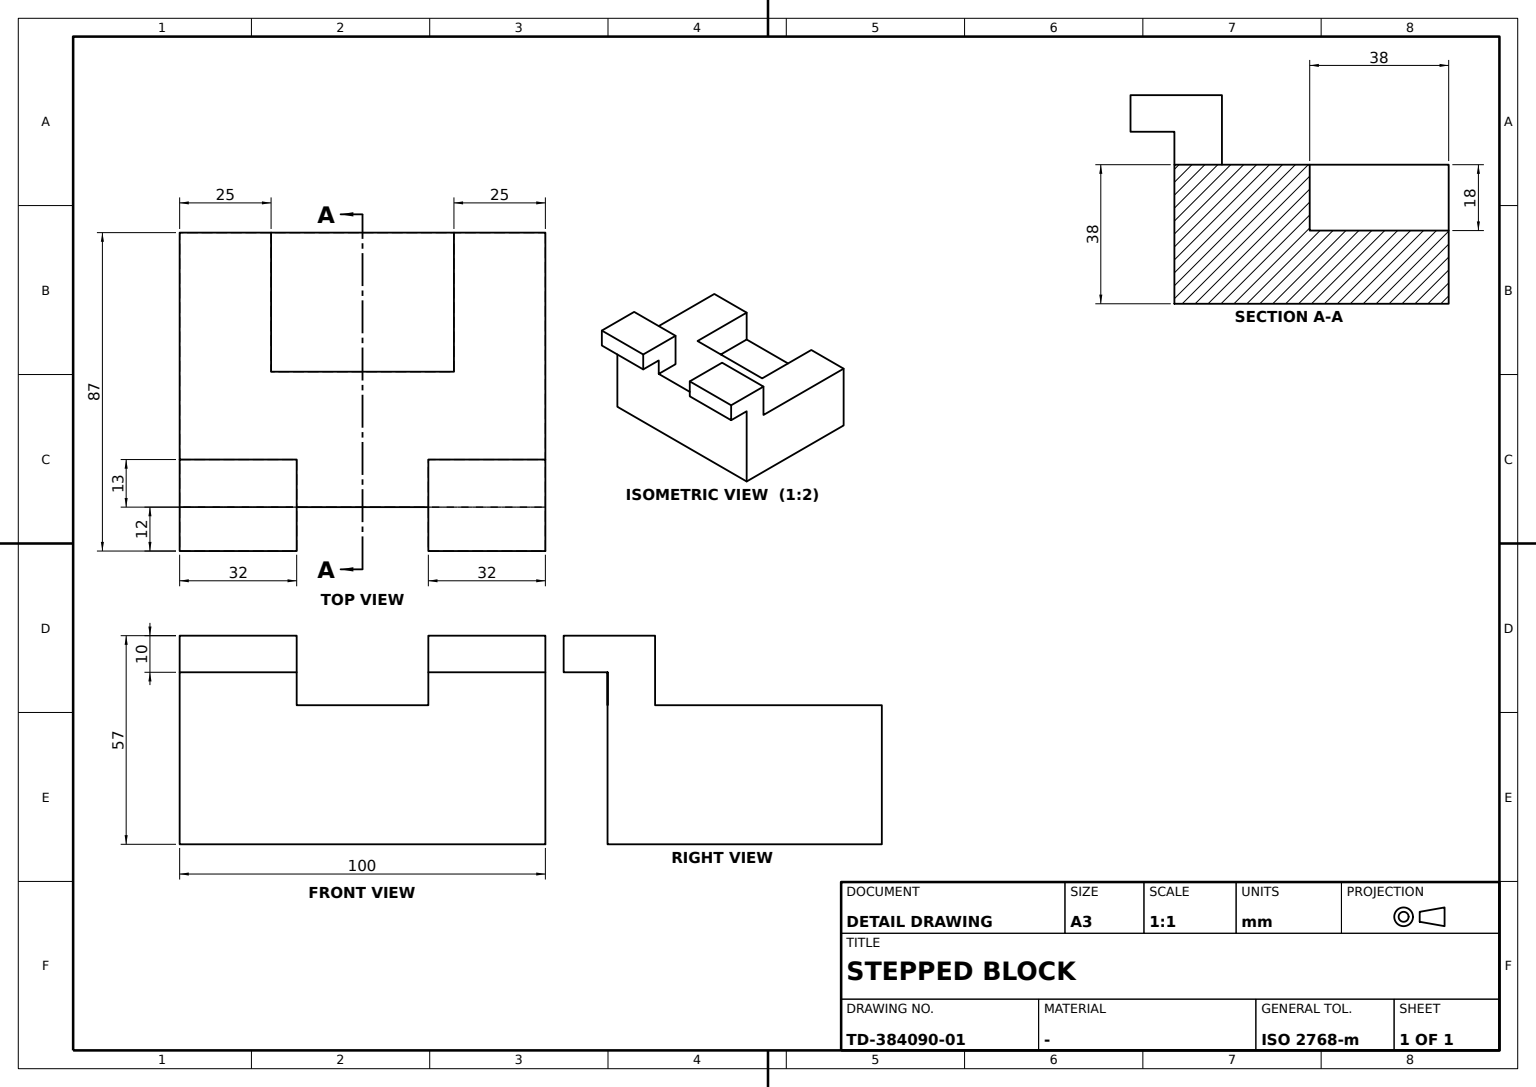
ISO-10303-21;
HEADER;
FILE_DESCRIPTION((''),'2;1');
FILE_NAME('','',(''),(''),'','','');
FILE_SCHEMA(('AUTOMOTIVE_DESIGN'));
ENDSEC;
DATA;
#1=APPLICATION_CONTEXT('');
#2=PRODUCT_CONTEXT('',#1,'mechanical');
#3=PRODUCT('','','',(#2));
#4=PRODUCT_DEFINITION_FORMATION('','',#3);
#5=PRODUCT_DEFINITION_CONTEXT('',#1,'design');
#6=PRODUCT_DEFINITION('','',#4,#5);
#7=PRODUCT_DEFINITION_SHAPE('','',#6);
#8=(LENGTH_UNIT()NAMED_UNIT(*)SI_UNIT(.MILLI.,.METRE.));
#9=(NAMED_UNIT(*)PLANE_ANGLE_UNIT()SI_UNIT($,.RADIAN.));
#10=(NAMED_UNIT(*)SI_UNIT($,.STERADIAN.)SOLID_ANGLE_UNIT());
#11=UNCERTAINTY_MEASURE_WITH_UNIT(LENGTH_MEASURE(0.005),#8,'distance_accuracy_value','');
#12=(GEOMETRIC_REPRESENTATION_CONTEXT(3)GLOBAL_UNCERTAINTY_ASSIGNED_CONTEXT((#11))GLOBAL_UNIT_ASSIGNED_CONTEXT((#8,#9,#10))REPRESENTATION_CONTEXT('',''));
#13=CARTESIAN_POINT('',(-50.,-49.5,57.));
#14=VERTEX_POINT('',#13);
#15=CARTESIAN_POINT('',(-50.,-49.5,47.));
#16=VERTEX_POINT('',#15);
#17=DIRECTION('',(0.,0.,-1.));
#18=VECTOR('',#17,1000.);
#19=LINE('',#13,#18);
#20=EDGE_CURVE('',#14,#16,#19,.T.);
#21=ORIENTED_EDGE('',*,*,#20,.T.);
#22=CARTESIAN_POINT('',(-18.,-49.5,47.));
#23=VERTEX_POINT('',#22);
#24=CARTESIAN_POINT('',(50.,-49.5,47.));
#25=DIRECTION('',(1.,0.,0.));
#26=VECTOR('',#25,1000.);
#27=LINE('',#24,#26);
#28=EDGE_CURVE('',#16,#23,#27,.T.);
#29=ORIENTED_EDGE('',*,*,#28,.T.);
#30=CARTESIAN_POINT('',(-18.,-49.5,57.));
#31=VERTEX_POINT('',#30);
#32=LINE('',#30,#18);
#33=EDGE_CURVE('',#31,#23,#32,.T.);
#34=ORIENTED_EDGE('',*,*,#33,.F.);
#35=CARTESIAN_POINT('',(50.,-49.5,57.));
#36=LINE('',#35,#26);
#37=EDGE_CURVE('',#14,#31,#36,.T.);
#38=ORIENTED_EDGE('',*,*,#37,.F.);
#39=EDGE_LOOP('',(#21,#29,#34,#38));
#40=FACE_BOUND('',#39,.T.);
#41=DIRECTION('',(0.,1.,0.));
#42=AXIS2_PLACEMENT_3D('',#35,#41,#17);
#43=PLANE('',#42);
#44=ADVANCED_FACE('',(#40),#43,.F.);
#45=CARTESIAN_POINT('',(-50.,-37.5,47.));
#46=VERTEX_POINT('',#45);
#47=CARTESIAN_POINT('',(-18.,-37.5,47.));
#48=VERTEX_POINT('',#47);
#49=CARTESIAN_POINT('',(50.,-37.5,47.));
#50=LINE('',#49,#26);
#51=EDGE_CURVE('',#46,#48,#50,.T.);
#52=ORIENTED_EDGE('',*,*,#51,.T.);
#53=VECTOR('',#41,1000.);
#54=LINE('',#22,#53);
#55=EDGE_CURVE('',#23,#48,#54,.T.);
#56=ORIENTED_EDGE('',*,*,#55,.F.);
#57=ORIENTED_EDGE('',*,*,#28,.F.);
#58=LINE('',#15,#53);
#59=EDGE_CURVE('',#16,#46,#58,.T.);
#60=ORIENTED_EDGE('',*,*,#59,.T.);
#61=EDGE_LOOP('',(#52,#56,#57,#60));
#62=FACE_BOUND('',#61,.T.);
#63=DIRECTION('',(0.,0.,1.));
#64=AXIS2_PLACEMENT_3D('',#24,#63,#41);
#65=PLANE('',#64);
#66=ADVANCED_FACE('',(#62),#65,.F.);
#67=CARTESIAN_POINT('',(-50.,-37.5,0.));
#68=VERTEX_POINT('',#67);
#69=VECTOR('',#63,1000.);
#70=LINE('',#67,#69);
#71=EDGE_CURVE('',#68,#46,#70,.T.);
#72=ORIENTED_EDGE('',*,*,#71,.F.);
#73=CARTESIAN_POINT('',(50.,-37.5,0.));
#74=VERTEX_POINT('',#73);
#75=CARTESIAN_POINT('',(0.,-37.5,0.));
#76=DIRECTION('',(-1.,0.,0.));
#77=VECTOR('',#76,1000.);
#78=LINE('',#75,#77);
#79=EDGE_CURVE('',#74,#68,#78,.T.);
#80=ORIENTED_EDGE('',*,*,#79,.F.);
#81=VERTEX_POINT('',#49);
#82=LINE('',#73,#69);
#83=EDGE_CURVE('',#74,#81,#82,.T.);
#84=ORIENTED_EDGE('',*,*,#83,.T.);
#85=CARTESIAN_POINT('',(18.,-37.5,47.));
#86=VERTEX_POINT('',#85);
#87=LINE('',#49,#77);
#88=EDGE_CURVE('',#81,#86,#87,.T.);
#89=ORIENTED_EDGE('',*,*,#88,.T.);
#90=CARTESIAN_POINT('',(18.,-37.5,38.));
#91=VERTEX_POINT('',#90);
#92=CARTESIAN_POINT('',(18.,-37.5,0.));
#93=LINE('',#92,#18);
#94=EDGE_CURVE('',#86,#91,#93,.T.);
#95=ORIENTED_EDGE('',*,*,#94,.T.);
#96=CARTESIAN_POINT('',(-18.,-37.5,38.));
#97=VERTEX_POINT('',#96);
#98=CARTESIAN_POINT('',(0.,-37.5,38.));
#99=LINE('',#98,#77);
#100=EDGE_CURVE('',#91,#97,#99,.T.);
#101=ORIENTED_EDGE('',*,*,#100,.T.);
#102=CARTESIAN_POINT('',(-18.,-37.5,0.));
#103=LINE('',#102,#18);
#104=EDGE_CURVE('',#48,#97,#103,.T.);
#105=ORIENTED_EDGE('',*,*,#104,.F.);
#106=ORIENTED_EDGE('',*,*,#51,.F.);
#107=EDGE_LOOP('',(#72,#80,#84,#89,#95,#101,#105,#106));
#108=FACE_BOUND('',#107,.T.);
#109=AXIS2_PLACEMENT_3D('',#73,#41,#76);
#110=PLANE('',#109);
#111=ADVANCED_FACE('',(#108),#110,.F.);
#112=CARTESIAN_POINT('',(18.,-24.5,57.));
#113=VERTEX_POINT('',#112);
#114=CARTESIAN_POINT('',(18.,-49.5,57.));
#115=VERTEX_POINT('',#114);
#116=DIRECTION('',(0.,-1.,0.));
#117=VECTOR('',#116,1000.);
#118=LINE('',#112,#117);
#119=EDGE_CURVE('',#113,#115,#118,.T.);
#120=ORIENTED_EDGE('',*,*,#119,.T.);
#121=VERTEX_POINT('',#35);
#122=LINE('',#35,#77);
#123=EDGE_CURVE('',#121,#115,#122,.T.);
#124=ORIENTED_EDGE('',*,*,#123,.F.);
#125=CARTESIAN_POINT('',(50.,-24.5,57.));
#126=VERTEX_POINT('',#125);
#127=CARTESIAN_POINT('',(50.,37.5,57.));
#128=LINE('',#127,#117);
#129=EDGE_CURVE('',#126,#121,#128,.T.);
#130=ORIENTED_EDGE('',*,*,#129,.F.);
#131=LINE('',#125,#77);
#132=EDGE_CURVE('',#126,#113,#131,.T.);
#133=ORIENTED_EDGE('',*,*,#132,.T.);
#134=EDGE_LOOP('',(#120,#124,#130,#133));
#135=FACE_BOUND('',#134,.T.);
#136=AXIS2_PLACEMENT_3D('',#125,#17,#116);
#137=PLANE('',#136);
#138=ADVANCED_FACE('',(#135),#137,.F.);
#139=CARTESIAN_POINT('',(25.,-0.5,38.));
#140=VERTEX_POINT('',#139);
#141=CARTESIAN_POINT('',(25.,-0.5,20.));
#142=VERTEX_POINT('',#141);
#143=LINE('',#139,#18);
#144=EDGE_CURVE('',#140,#142,#143,.T.);
#145=ORIENTED_EDGE('',*,*,#144,.T.);
#146=CARTESIAN_POINT('',(-25.,-0.5,20.));
#147=VERTEX_POINT('',#146);
#148=LINE('',#146,#26);
#149=EDGE_CURVE('',#147,#142,#148,.T.);
#150=ORIENTED_EDGE('',*,*,#149,.F.);
#151=CARTESIAN_POINT('',(-25.,-0.5,38.));
#152=VERTEX_POINT('',#151);
#153=LINE('',#151,#18);
#154=EDGE_CURVE('',#152,#147,#153,.T.);
#155=ORIENTED_EDGE('',*,*,#154,.F.);
#156=LINE('',#151,#26);
#157=EDGE_CURVE('',#152,#140,#156,.T.);
#158=ORIENTED_EDGE('',*,*,#157,.T.);
#159=EDGE_LOOP('',(#145,#150,#155,#158));
#160=FACE_BOUND('',#159,.T.);
#161=AXIS2_PLACEMENT_3D('',#151,#41,#25);
#162=PLANE('',#161);
#163=ADVANCED_FACE('',(#160),#162,.T.);
#164=CARTESIAN_POINT('',(25.,37.5,38.));
#165=VERTEX_POINT('',#164);
#166=LINE('',#139,#53);
#167=EDGE_CURVE('',#140,#165,#166,.T.);
#168=ORIENTED_EDGE('',*,*,#167,.F.);
#169=ORIENTED_EDGE('',*,*,#157,.F.);
#170=CARTESIAN_POINT('',(-25.,37.5,38.));
#171=VERTEX_POINT('',#170);
#172=LINE('',#170,#117);
#173=EDGE_CURVE('',#171,#152,#172,.T.);
#174=ORIENTED_EDGE('',*,*,#173,.F.);
#175=CARTESIAN_POINT('',(-50.,37.5,38.));
#176=VERTEX_POINT('',#175);
#177=CARTESIAN_POINT('',(0.,37.5,38.));
#178=LINE('',#177,#26);
#179=EDGE_CURVE('',#176,#171,#178,.T.);
#180=ORIENTED_EDGE('',*,*,#179,.F.);
#181=CARTESIAN_POINT('',(-50.,-24.5,38.));
#182=VERTEX_POINT('',#181);
#183=CARTESIAN_POINT('',(-50.,0.,38.));
#184=LINE('',#183,#53);
#185=EDGE_CURVE('',#182,#176,#184,.T.);
#186=ORIENTED_EDGE('',*,*,#185,.F.);
#187=CARTESIAN_POINT('',(-18.,-24.5,38.));
#188=VERTEX_POINT('',#187);
#189=CARTESIAN_POINT('',(0.,-24.5,38.));
#190=LINE('',#189,#26);
#191=EDGE_CURVE('',#182,#188,#190,.T.);
#192=ORIENTED_EDGE('',*,*,#191,.T.);
#193=CARTESIAN_POINT('',(-18.,0.,38.));
#194=LINE('',#193,#53);
#195=EDGE_CURVE('',#97,#188,#194,.T.);
#196=ORIENTED_EDGE('',*,*,#195,.F.);
#197=ORIENTED_EDGE('',*,*,#100,.F.);
#198=CARTESIAN_POINT('',(18.,-24.5,38.));
#199=VERTEX_POINT('',#198);
#200=CARTESIAN_POINT('',(18.,0.,38.));
#201=LINE('',#200,#53);
#202=EDGE_CURVE('',#91,#199,#201,.T.);
#203=ORIENTED_EDGE('',*,*,#202,.T.);
#204=CARTESIAN_POINT('',(50.,-24.5,38.));
#205=VERTEX_POINT('',#204);
#206=LINE('',#204,#77);
#207=EDGE_CURVE('',#205,#199,#206,.T.);
#208=ORIENTED_EDGE('',*,*,#207,.F.);
#209=CARTESIAN_POINT('',(50.,37.5,38.));
#210=VERTEX_POINT('',#209);
#211=CARTESIAN_POINT('',(50.,0.,38.));
#212=LINE('',#211,#117);
#213=EDGE_CURVE('',#210,#205,#212,.T.);
#214=ORIENTED_EDGE('',*,*,#213,.F.);
#215=EDGE_CURVE('',#165,#210,#178,.T.);
#216=ORIENTED_EDGE('',*,*,#215,.F.);
#217=EDGE_LOOP('',(#168,#169,#174,#180,#186,#192,#196,#197,#203,#208,#214,#216));
#218=FACE_BOUND('',#217,.T.);
#219=CARTESIAN_POINT('',(0.,0.,38.));
#220=AXIS2_PLACEMENT_3D('',#219,#63,#25);
#221=PLANE('',#220);
#222=ADVANCED_FACE('',(#218),#221,.T.);
#223=ORIENTED_EDGE('',*,*,#173,.T.);
#224=ORIENTED_EDGE('',*,*,#154,.T.);
#225=CARTESIAN_POINT('',(-25.,37.5,20.));
#226=VERTEX_POINT('',#225);
#227=LINE('',#225,#117);
#228=EDGE_CURVE('',#226,#147,#227,.T.);
#229=ORIENTED_EDGE('',*,*,#228,.F.);
#230=LINE('',#170,#18);
#231=EDGE_CURVE('',#171,#226,#230,.T.);
#232=ORIENTED_EDGE('',*,*,#231,.F.);
#233=EDGE_LOOP('',(#223,#224,#229,#232));
#234=FACE_BOUND('',#233,.T.);
#235=AXIS2_PLACEMENT_3D('',#170,#25,#116);
#236=PLANE('',#235);
#237=ADVANCED_FACE('',(#234),#236,.T.);
#238=CARTESIAN_POINT('',(25.,37.5,20.));
#239=VERTEX_POINT('',#238);
#240=LINE('',#141,#53);
#241=EDGE_CURVE('',#142,#239,#240,.T.);
#242=ORIENTED_EDGE('',*,*,#241,.F.);
#243=ORIENTED_EDGE('',*,*,#144,.F.);
#244=ORIENTED_EDGE('',*,*,#167,.T.);
#245=CARTESIAN_POINT('',(25.,37.5,0.));
#246=LINE('',#245,#18);
#247=EDGE_CURVE('',#165,#239,#246,.T.);
#248=ORIENTED_EDGE('',*,*,#247,.T.);
#249=EDGE_LOOP('',(#242,#243,#244,#248));
#250=FACE_BOUND('',#249,.T.);
#251=AXIS2_PLACEMENT_3D('',#139,#76,#41);
#252=PLANE('',#251);
#253=ADVANCED_FACE('',(#250),#252,.T.);
#254=ORIENTED_EDGE('',*,*,#129,.T.);
#255=VERTEX_POINT('',#24);
#256=CARTESIAN_POINT('',(50.,-49.5,0.));
#257=LINE('',#256,#18);
#258=EDGE_CURVE('',#121,#255,#257,.T.);
#259=ORIENTED_EDGE('',*,*,#258,.T.);
#260=CARTESIAN_POINT('',(50.,37.5,47.));
#261=LINE('',#260,#53);
#262=EDGE_CURVE('',#255,#81,#261,.T.);
#263=ORIENTED_EDGE('',*,*,#262,.T.);
#264=ORIENTED_EDGE('',*,*,#83,.F.);
#265=CARTESIAN_POINT('',(50.,37.5,0.));
#266=VERTEX_POINT('',#265);
#267=CARTESIAN_POINT('',(50.,0.,0.));
#268=LINE('',#267,#117);
#269=EDGE_CURVE('',#266,#74,#268,.T.);
#270=ORIENTED_EDGE('',*,*,#269,.F.);
#271=LINE('',#265,#69);
#272=EDGE_CURVE('',#266,#210,#271,.T.);
#273=ORIENTED_EDGE('',*,*,#272,.T.);
#274=ORIENTED_EDGE('',*,*,#213,.T.);
#275=CARTESIAN_POINT('',(50.,-24.5,0.));
#276=LINE('',#275,#69);
#277=EDGE_CURVE('',#205,#126,#276,.T.);
#278=ORIENTED_EDGE('',*,*,#277,.T.);
#279=EDGE_LOOP('',(#254,#259,#263,#264,#270,#273,#274,#278));
#280=FACE_BOUND('',#279,.T.);
#281=AXIS2_PLACEMENT_3D('',#265,#76,#116);
#282=PLANE('',#281);
#283=ADVANCED_FACE('',(#280),#282,.F.);
#284=CARTESIAN_POINT('',(-50.,-24.5,57.));
#285=VERTEX_POINT('',#284);
#286=LINE('',#284,#117);
#287=EDGE_CURVE('',#285,#14,#286,.T.);
#288=ORIENTED_EDGE('',*,*,#287,.T.);
#289=ORIENTED_EDGE('',*,*,#37,.T.);
#290=CARTESIAN_POINT('',(-18.,-24.5,57.));
#291=VERTEX_POINT('',#290);
#292=LINE('',#290,#117);
#293=EDGE_CURVE('',#291,#31,#292,.T.);
#294=ORIENTED_EDGE('',*,*,#293,.F.);
#295=LINE('',#125,#26);
#296=EDGE_CURVE('',#285,#291,#295,.T.);
#297=ORIENTED_EDGE('',*,*,#296,.F.);
#298=EDGE_LOOP('',(#288,#289,#294,#297));
#299=FACE_BOUND('',#298,.T.);
#300=ADVANCED_FACE('',(#299),#137,.F.);
#301=LINE('',#181,#69);
#302=EDGE_CURVE('',#182,#285,#301,.T.);
#303=ORIENTED_EDGE('',*,*,#302,.T.);
#304=ORIENTED_EDGE('',*,*,#296,.T.);
#305=LINE('',#187,#69);
#306=EDGE_CURVE('',#188,#291,#305,.T.);
#307=ORIENTED_EDGE('',*,*,#306,.F.);
#308=ORIENTED_EDGE('',*,*,#191,.F.);
#309=EDGE_LOOP('',(#303,#304,#307,#308));
#310=FACE_BOUND('',#309,.T.);
#311=AXIS2_PLACEMENT_3D('',#204,#116,#63);
#312=PLANE('',#311);
#313=ADVANCED_FACE('',(#310),#312,.F.);
#314=ORIENTED_EDGE('',*,*,#302,.F.);
#315=ORIENTED_EDGE('',*,*,#185,.T.);
#316=CARTESIAN_POINT('',(-50.,37.5,0.));
#317=VERTEX_POINT('',#316);
#318=LINE('',#316,#69);
#319=EDGE_CURVE('',#317,#176,#318,.T.);
#320=ORIENTED_EDGE('',*,*,#319,.F.);
#321=CARTESIAN_POINT('',(-50.,0.,0.));
#322=LINE('',#321,#53);
#323=EDGE_CURVE('',#68,#317,#322,.T.);
#324=ORIENTED_EDGE('',*,*,#323,.F.);
#325=ORIENTED_EDGE('',*,*,#71,.T.);
#326=ORIENTED_EDGE('',*,*,#59,.F.);
#327=ORIENTED_EDGE('',*,*,#20,.F.);
#328=ORIENTED_EDGE('',*,*,#287,.F.);
#329=EDGE_LOOP('',(#314,#315,#320,#324,#325,#326,#327,#328));
#330=FACE_BOUND('',#329,.T.);
#331=AXIS2_PLACEMENT_3D('',#67,#25,#41);
#332=PLANE('',#331);
#333=ADVANCED_FACE('',(#330),#332,.F.);
#334=ORIENTED_EDGE('',*,*,#179,.T.);
#335=ORIENTED_EDGE('',*,*,#231,.T.);
#336=CARTESIAN_POINT('',(-50.,37.5,20.));
#337=LINE('',#336,#77);
#338=EDGE_CURVE('',#239,#226,#337,.T.);
#339=ORIENTED_EDGE('',*,*,#338,.F.);
#340=ORIENTED_EDGE('',*,*,#247,.F.);
#341=ORIENTED_EDGE('',*,*,#215,.T.);
#342=ORIENTED_EDGE('',*,*,#272,.F.);
#343=CARTESIAN_POINT('',(0.,37.5,0.));
#344=LINE('',#343,#26);
#345=EDGE_CURVE('',#317,#266,#344,.T.);
#346=ORIENTED_EDGE('',*,*,#345,.F.);
#347=ORIENTED_EDGE('',*,*,#319,.T.);
#348=EDGE_LOOP('',(#334,#335,#339,#340,#341,#342,#346,#347));
#349=FACE_BOUND('',#348,.T.);
#350=AXIS2_PLACEMENT_3D('',#316,#116,#25);
#351=PLANE('',#350);
#352=ADVANCED_FACE('',(#349),#351,.F.);
#353=ORIENTED_EDGE('',*,*,#241,.T.);
#354=ORIENTED_EDGE('',*,*,#338,.T.);
#355=ORIENTED_EDGE('',*,*,#228,.T.);
#356=ORIENTED_EDGE('',*,*,#149,.T.);
#357=EDGE_LOOP('',(#353,#354,#355,#356));
#358=FACE_BOUND('',#357,.T.);
#359=CARTESIAN_POINT('',(0.,0.,20.));
#360=AXIS2_PLACEMENT_3D('',#359,#63,#25);
#361=PLANE('',#360);
#362=ADVANCED_FACE('',(#358),#361,.T.);
#363=ORIENTED_EDGE('',*,*,#323,.T.);
#364=ORIENTED_EDGE('',*,*,#345,.T.);
#365=ORIENTED_EDGE('',*,*,#269,.T.);
#366=ORIENTED_EDGE('',*,*,#79,.T.);
#367=EDGE_LOOP('',(#363,#364,#365,#366));
#368=FACE_BOUND('',#367,.T.);
#369=CARTESIAN_POINT('',(0.,0.,0.));
#370=AXIS2_PLACEMENT_3D('',#369,#63,#25);
#371=PLANE('',#370);
#372=ADVANCED_FACE('',(#368),#371,.F.);
#373=CARTESIAN_POINT('',(18.,-49.5,47.));
#374=VERTEX_POINT('',#373);
#375=LINE('',#24,#77);
#376=EDGE_CURVE('',#255,#374,#375,.T.);
#377=ORIENTED_EDGE('',*,*,#376,.F.);
#378=ORIENTED_EDGE('',*,*,#258,.F.);
#379=ORIENTED_EDGE('',*,*,#123,.T.);
#380=LINE('',#114,#18);
#381=EDGE_CURVE('',#115,#374,#380,.T.);
#382=ORIENTED_EDGE('',*,*,#381,.T.);
#383=EDGE_LOOP('',(#377,#378,#379,#382));
#384=FACE_BOUND('',#383,.T.);
#385=ADVANCED_FACE('',(#384),#43,.F.);
#386=LINE('',#373,#53);
#387=EDGE_CURVE('',#374,#86,#386,.T.);
#388=ORIENTED_EDGE('',*,*,#387,.F.);
#389=ORIENTED_EDGE('',*,*,#381,.F.);
#390=ORIENTED_EDGE('',*,*,#119,.F.);
#391=LINE('',#198,#69);
#392=EDGE_CURVE('',#199,#113,#391,.T.);
#393=ORIENTED_EDGE('',*,*,#392,.F.);
#394=ORIENTED_EDGE('',*,*,#202,.F.);
#395=ORIENTED_EDGE('',*,*,#94,.F.);
#396=EDGE_LOOP('',(#388,#389,#390,#393,#394,#395));
#397=FACE_BOUND('',#396,.T.);
#398=CARTESIAN_POINT('',(18.,0.,0.));
#399=AXIS2_PLACEMENT_3D('',#398,#25,#41);
#400=PLANE('',#399);
#401=ADVANCED_FACE('',(#397),#400,.F.);
#402=ORIENTED_EDGE('',*,*,#277,.F.);
#403=ORIENTED_EDGE('',*,*,#207,.T.);
#404=ORIENTED_EDGE('',*,*,#392,.T.);
#405=ORIENTED_EDGE('',*,*,#132,.F.);
#406=EDGE_LOOP('',(#402,#403,#404,#405));
#407=FACE_BOUND('',#406,.T.);
#408=ADVANCED_FACE('',(#407),#312,.F.);
#409=ORIENTED_EDGE('',*,*,#55,.T.);
#410=ORIENTED_EDGE('',*,*,#104,.T.);
#411=ORIENTED_EDGE('',*,*,#195,.T.);
#412=ORIENTED_EDGE('',*,*,#306,.T.);
#413=ORIENTED_EDGE('',*,*,#293,.T.);
#414=ORIENTED_EDGE('',*,*,#33,.T.);
#415=EDGE_LOOP('',(#409,#410,#411,#412,#413,#414));
#416=FACE_BOUND('',#415,.T.);
#417=CARTESIAN_POINT('',(-18.,0.,0.));
#418=AXIS2_PLACEMENT_3D('',#417,#25,#41);
#419=PLANE('',#418);
#420=ADVANCED_FACE('',(#416),#419,.T.);
#421=ORIENTED_EDGE('',*,*,#387,.T.);
#422=ORIENTED_EDGE('',*,*,#88,.F.);
#423=ORIENTED_EDGE('',*,*,#262,.F.);
#424=ORIENTED_EDGE('',*,*,#376,.T.);
#425=EDGE_LOOP('',(#421,#422,#423,#424));
#426=FACE_BOUND('',#425,.T.);
#427=ADVANCED_FACE('',(#426),#65,.F.);
#428=CLOSED_SHELL('',(#44,#66,#111,#138,#163,#222,#237,#253,#283,#300,#313,#333,#352,#362,#372,#385,#401,#408,#420,#427));
#429=MANIFOLD_SOLID_BREP('',#428);
#430=ADVANCED_BREP_SHAPE_REPRESENTATION('',(#429),#12);
#431=SHAPE_DEFINITION_REPRESENTATION(#7,#430);
ENDSEC;
END-ISO-10303-21;
